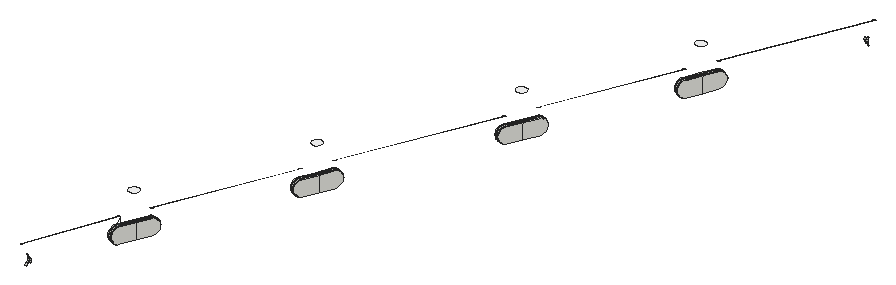
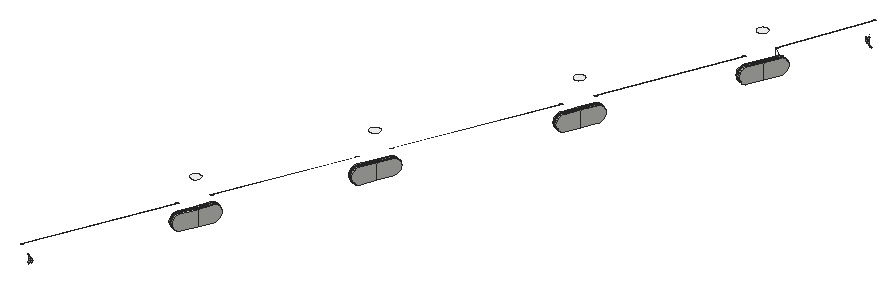
# SketchUp Ruby script. Lengths in inches.
U = 1.inch
M = Sketchup.active_model
def pt(a) = Geom::Point3d.new(a.map { |v| v * U })
def face(e, loops, mat)
  f = e.add_face(loops[0].map { |a| pt(a) })
  loops[1..].each { |l| e.add_face(l.map { |a| pt(a) }).erase! }
  f.material = f.back_material = mat if mat
  f
end
# faces: each face lists its corners as indices into pts; further lists are holes
def faces(e, pts, list, mat = nil) = list.each { |f| face(e, (f[0].is_a?(Array) ? f : [f]).map { |l| l.map { |i| pts[i] } }, mat) }
# xy, xz, yz: faces in a plane at the given z, y or x. An outline is a flat list of corners, or four numbers for a rectangle; further outlines are holes
def ring(l) = l.size == 4 ? [[l[0], l[1]], [l[2], l[1]], [l[2], l[3]], [l[0], l[3]]] : l.each_slice(2).to_a
def flat(e, list, mat, &to3) = list.each { |f| face(e, (f[0].is_a?(Array) ? f : [f]).map { |l| ring(l).map { |u, v| to3.(u, v) } }, mat) }
def xy(e, z, list, mat = nil) = flat(e, list, mat) { |x, y| [x, y, z] }
def xz(e, y, list, mat = nil) = flat(e, list, mat) { |x, z| [x, y, z] }
def yz(e, x, list, mat = nil) = flat(e, list, mat) { |y, z| [x, y, z] }
def lines(e, pts, list) = list.each { |a, b| e.add_line(pt(pts[a]), pt(pts[b])) }
# prism: a flat outline (further loops are holes) pulled along v
def prism(e, loops, v, mat = nil)
  f = face(e, loops, mat); d = Geom::Vector3d.new(v.map { |x| x * U })
  f.pushpull(f.normal.samedirection?(d) ? d.length : -d.length)
end
def box(e, o, s, mat = nil) = prism(e, [[o, [o[0] + s[0], o[1], o[2]], [o[0] + s[0], o[1] + s[1], o[2]], [o[0], o[1] + s[1], o[2]]]], [0, 0, s[2]], mat)
def at(x, y, z, deg = 0) = Geom::Transformation.translation(pt([x, y, z])) * Geom::Transformation.rotation(ORIGIN, Z_AXIS, deg.degrees)
def axes(o, x, y, z) = Geom::Transformation.new([*x, 0, *y, 0, *z, 0, *pt(o).to_a, 1])
def part(name) = M.definitions.add(name)
# library, detail: a bought-in or finely detailed component or shape, given as its bounding box
def library(name, o, s) = part(name).tap { |d| box(d.entities, o, s) }
def detail(e, o, s) = box(e.add_group.entities, o, s)
def put(e, d, t, mat = nil) = e.add_instance(d, t).tap { |i| i.material = mat if mat }
def group(e, t, mat = nil) = e.add_group.tap { |g| g.transformation = t; g.material = mat if mat }.entities
root = M.entities
M.materials.add("Glass_Safety_01").color = [204, 235, 244]
M.materials["Glass_Safety_01"].alpha = 0.1
M.materials.add("[Color_000]").color = [255, 255, 255]
xy(root,351.283,[[888.84,639.54,888.584,639.641,888.672,639.866,889.306,641.468,889.558,641.358],[888.4,639.713,888.144,639.814,888.868,641.645,889.124,641.544,888.489,639.938],[889.558,641.358,889.306,641.468,889.307,641.472,889.563,641.37,889.561,641.364],[889.563,641.37,889.307,641.472,890.092,643.273,890.344,643.163],[889.125,641.547,888.873,641.657,889.659,643.462,889.911,643.352],
  [897.674,659.993,897.421,660.103,897.491,660.262,898.207,661.907,898.46,661.797],[897.241,660.181,896.988,660.291,897.774,662.096,898.027,661.986,897.31,660.341],[898.46,661.797,898.207,661.907,898.994,663.712,899.246,663.602],[898.027,661.986,897.774,662.096,898.56,663.901,898.813,663.791],[907.619,682.827,907.367,682.937,907.429,683.08,908.153,684.742,908.405,684.632],
  [907.186,683.016,906.933,683.126,907.719,684.93,907.972,684.82,907.248,683.158],[908.405,684.632,908.153,684.742,908.939,686.547,909.191,686.436],[907.972,684.82,907.719,684.93,908.505,686.735,908.758,686.625],[916.339,702.848,916.086,702.958,916.157,703.12,916.872,704.763,917.125,704.653],[915.906,703.036,915.653,703.146,916.439,704.951,916.692,704.841,915.977,703.199],
  [917.125,704.653,916.872,704.763,917.658,706.567,917.911,706.457],[916.692,704.841,916.439,704.951,917.225,706.756,917.478,706.646]])
xy(root,351.362,[[888.728,640.007,888.545,640.079,889.124,641.544,889.215,641.508,889.306,641.468],[889.306,641.468,889.215,641.508,889.307,641.472,889.306,641.47],[889.307,641.472,889.215,641.508,889.125,641.547,889.754,642.991,889.935,642.912],[897.579,660.464,897.398,660.542,898.027,661.986,898.207,661.907],[898.207,661.907,898.027,661.986,898.656,663.43,898.836,663.351],
  [907.524,683.298,907.343,683.377,907.972,684.82,908.153,684.742],[908.153,684.742,907.972,684.82,908.601,686.264,908.781,686.186],[916.243,703.319,916.063,703.397,916.692,704.841,916.872,704.763],[916.872,704.763,916.692,704.841,917.321,706.285,917.501,706.206]],"Glass_Safety_01")
xy(root,353.33,[[888.728,640.007,889.306,641.468,889.215,641.508,889.124,641.544,888.545,640.079],[889.306,641.468,889.306,641.47,889.307,641.472,889.215,641.508],[889.307,641.472,889.935,642.912,889.754,642.991,889.125,641.547,889.215,641.508],[897.579,660.464,898.207,661.907,898.027,661.986,897.398,660.542],[898.207,661.907,898.836,663.351,898.656,663.43,898.027,661.986],
  [907.524,683.298,908.153,684.742,907.972,684.82,907.343,683.377],[908.153,684.742,908.781,686.186,908.601,686.264,907.972,684.82],[916.243,703.319,916.872,704.763,916.692,704.841,916.063,703.397],[916.872,704.763,917.501,706.206,917.321,706.285,916.692,704.841]],"Glass_Safety_01")
xy(root,353.409,[[888.84,639.54,889.558,641.358,889.306,641.468,888.672,639.866,888.584,639.641],[888.4,639.713,888.489,639.938,889.124,641.544,888.868,641.645,888.144,639.814],[889.558,641.358,889.561,641.364,889.563,641.37,889.307,641.472,889.306,641.468],[889.563,641.37,890.344,643.163,890.092,643.273,889.307,641.472],[889.125,641.547,889.911,643.352,889.659,643.462,888.873,641.657],
  [897.674,659.993,898.46,661.797,898.207,661.907,897.491,660.262,897.421,660.103],[897.241,660.181,897.31,660.341,898.027,661.986,897.774,662.096,896.988,660.291],[898.46,661.797,899.246,663.602,898.994,663.712,898.207,661.907],[898.027,661.986,898.813,663.791,898.56,663.901,897.774,662.096],[907.619,682.827,908.405,684.632,908.153,684.742,907.429,683.08,907.367,682.937],
  [907.186,683.016,907.248,683.158,907.972,684.82,907.719,684.93,906.933,683.126],[908.405,684.632,909.191,686.436,908.939,686.547,908.153,684.742],[907.972,684.82,908.758,686.625,908.505,686.735,907.719,684.93],[916.339,702.848,917.125,704.653,916.872,704.763,916.157,703.12,916.086,702.958],[915.906,703.036,915.977,703.199,916.692,704.841,916.439,704.951,915.653,703.146],
  [917.125,704.653,917.911,706.457,917.658,706.567,916.872,704.763],[916.692,704.841,917.478,706.646,917.225,706.756,916.439,704.951]])
xy(root,354.511,[[884.14,628.396,888.489,639.938,883.957,628.468],[884.14,628.396,888.672,639.866,888.489,639.938],[890.092,643.273,897.31,660.341,889.911,643.352],[890.092,643.273,897.491,660.262,897.31,660.341],[898.994,663.712,907.248,683.158,898.813,663.791],
  [898.994,663.712,907.429,683.08,907.248,683.158],[908.939,686.547,915.977,703.199,908.758,686.625],[908.939,686.547,916.157,703.12,915.977,703.199],[917.658,706.567,925.204,724.386,917.478,706.646],[917.658,706.567,925.385,724.307,925.204,724.386]],"Glass_Safety_01")
xy(root,357.267,[[889.26,640.879,889.422,640.912,889.569,640.986,889.692,641.095,889.782,641.233,889.834,641.389,889.844,641.553,889.811,641.714,889.737,641.861,889.628,641.984,889.491,642.074,889.335,642.126,889.17,642.136,889.009,642.103,888.862,642.029,888.739,641.92,888.649,641.783,888.597,641.627,888.587,641.463,888.62,641.302,888.694,641.155,888.803,641.032,888.94,640.941,889.096,640.889],[898.162,661.318,898.323,661.351,898.47,661.425,898.593,661.534,898.684,661.672,898.736,661.828,898.746,661.992,898.712,662.153,898.639,662.3,898.53,662.423,898.392,662.513,898.236,662.565,898.072,662.575,897.911,662.542,897.764,662.468,897.641,662.359,897.551,662.222,897.499,662.066,897.489,661.902,897.522,661.741,897.596,661.594,897.705,661.471,897.842,661.38,897.998,661.328],[908.107,684.153,908.268,684.186,908.415,684.259,908.538,684.369,908.629,684.506,908.681,684.662,908.691,684.826,908.658,684.987,908.584,685.134,908.475,685.257,908.337,685.348,908.181,685.4,908.017,685.409,907.856,685.376,907.709,685.303,907.586,685.194,907.496,685.056,907.444,684.9,907.434,684.736,907.467,684.575,907.541,684.428,907.65,684.305,907.787,684.214,907.943,684.163],[916.827,704.174,916.988,704.207,917.135,704.28,917.258,704.389,917.349,704.527,917.4,704.683,917.41,704.847,917.377,705.008,917.304,705.155,917.194,705.278,917.057,705.368,916.901,705.42,916.737,705.43,916.576,705.397,916.429,705.323,916.306,705.214,916.215,705.077,916.163,704.921,916.154,704.757,916.187,704.596,916.26,704.449,916.37,704.326,916.507,704.235,916.663,704.183]],"[Color_000]")
p = [[888.84,639.54,351.283],[889.558,641.358,351.283],[889.558,641.358,353.409],[888.84,639.54,353.409],[888.739,639.284,353.373],[888.644,639.045,353.267],
  [888.564,638.84,353.098],[888.501,638.683,352.877],[888.462,638.585,352.621],[888.449,638.551,352.346],[888.462,638.585,352.071],[888.501,638.683,351.814],
  [888.564,638.84,351.594],[888.644,639.045,351.425],[888.739,639.284,351.319],[888.4,639.713,351.283],[888.489,639.938,351.283],[888.489,639.938,353.409],
  [888.4,639.713,353.409],[888.299,639.457,353.373],[888.205,639.219,353.267],[888.124,639.014,353.098],[888.062,638.857,352.877],[888.023,638.758,352.621],
  [888.01,638.725,352.346],[888.023,638.758,352.071],[888.062,638.857,351.814],[888.124,639.014,351.594],[888.205,639.219,351.425],[888.299,639.457,351.319],
  [888.433,639.26,353.317],[888.202,638.675,352.163],[888.206,638.686,352.071],[888.245,638.785,351.814],[888.307,638.942,351.594],[888.388,639.147,351.425],
  [888.482,639.385,351.319],[888.584,639.641,351.283],[888.672,639.866,351.283],[888.672,639.866,353.409],[888.672,639.866,354.511],[889.306,641.468,353.409],
  [889.306,641.468,353.33],[889.306,641.468,351.362],[889.306,641.468,351.283],[888.193,638.652,352.346],[888.206,638.686,352.621],[888.245,638.785,352.877],
  [888.307,638.942,353.098],[888.388,639.147,353.267],[888.482,639.385,353.373],[888.584,639.641,353.409],[888.144,639.814,353.409],[888.868,641.645,353.409],
  [888.868,641.645,351.283],[888.144,639.814,351.283],[888.043,639.559,351.319],[887.949,639.32,351.425],[887.868,639.115,351.594],[887.806,638.958,351.814],
  [887.767,638.86,352.071],[887.753,638.826,352.346],[887.767,638.86,352.621],[887.806,638.958,352.877],[887.868,639.115,353.098],[887.949,639.32,353.267],
  [888.043,639.559,353.373],[889.124,641.544,353.409],[889.124,641.544,351.283],[889.124,641.544,351.362],[888.545,640.079,351.362],[888.545,640.079,353.33],
  [889.124,641.544,353.33],[889.307,641.472,351.283],[889.307,641.472,351.362],[889.307,641.472,353.33],[889.307,641.472,353.409],[889.563,641.37,353.409],
  [889.563,641.37,351.283],[889.561,641.364,353.409],[889.561,641.364,351.283],[890.344,643.163,351.283],[890.454,643.415,351.319],[890.557,643.65,351.425],
  [890.645,643.852,351.594],[890.712,644.007,351.814],[890.754,644.105,352.071],[890.769,644.138,352.346],[890.754,644.105,352.621],[890.712,644.007,352.877],
  [890.645,643.852,353.098],[890.557,643.65,353.267],[890.454,643.415,353.373],[890.344,643.163,353.409],[889.125,641.547,351.283],[889.125,641.547,351.362],
  [889.125,641.547,353.33],[889.125,641.547,353.409],[888.873,641.657,353.409],[888.873,641.657,351.283],[889.911,643.352,351.283],[889.911,643.352,353.409],
  [889.754,642.991,353.33],[889.754,642.991,351.362],[890.092,643.273,353.409],[890.202,643.525,353.373],[890.304,643.76,353.267],[890.392,643.962,353.098],
  [890.459,644.117,352.877],[890.502,644.215,352.621],[890.516,644.248,352.346],[890.502,644.215,352.071],[890.459,644.117,351.814],[890.392,643.962,351.594],
  [890.304,643.76,351.425],[890.202,643.525,351.319],[890.092,643.273,351.283],[889.659,643.462,353.409],[889.768,643.714,353.373],[889.871,643.949,353.267],
  [889.959,644.151,353.098],[890.026,644.306,352.877],[890.069,644.403,352.621],[890.083,644.436,352.346],[890.069,644.403,352.071],[890.026,644.306,351.814],
  [889.959,644.151,351.594],[889.871,643.949,351.425],[889.768,643.714,351.319],[889.659,643.462,351.283],[890.021,643.604,351.319],[890.021,643.604,353.373],
  [890.123,643.839,353.267],[890.211,644.041,353.098],[890.279,644.196,352.877],[890.321,644.293,352.621],[890.336,644.326,352.346],[890.321,644.293,352.071],
  [890.279,644.196,351.814],[890.211,644.041,351.594],[890.123,643.839,351.425],[898.46,661.797,353.409],[897.674,659.993,353.409],[897.564,659.74,353.373],
  [897.462,659.505,353.267],[897.374,659.303,353.098],[897.307,659.149,352.877],[897.264,659.051,352.621],[897.25,659.018,352.346],[897.264,659.051,352.071],
  [897.307,659.149,351.814],[897.374,659.303,351.594],[897.462,659.505,351.425],[897.564,659.74,351.319],[897.674,659.993,351.283],[898.46,661.797,351.283],
  [897.421,660.103,353.409],[897.491,660.262,353.409],[897.491,660.262,351.283],[897.421,660.103,351.283],[897.312,659.85,351.319],[897.209,659.615,351.425],
  [897.121,659.414,351.594],[897.054,659.259,351.814],[897.011,659.161,352.071],[896.997,659.128,352.346],[897.011,659.161,352.621],[897.054,659.259,352.877],
  [897.121,659.414,353.098],[897.209,659.615,353.267],[897.312,659.85,353.373],[897.241,660.181,351.283],[897.31,660.341,351.283],[897.31,660.341,353.409],
  [897.241,660.181,353.409],[897.131,659.929,353.373],[897.029,659.694,353.267],[896.941,659.492,353.098],[896.873,659.337,352.877],[896.831,659.24,352.621],
  [896.817,659.207,352.346],[896.831,659.24,352.071],[896.873,659.337,351.814],[896.941,659.492,351.594],[897.029,659.694,351.425],[897.131,659.929,351.319],
  [896.988,660.291,353.409],[897.774,662.096,353.409],[897.774,662.096,351.283],[896.988,660.291,351.283],[896.878,660.039,351.319],[896.776,659.804,351.425],
  [896.688,659.602,351.594],[896.621,659.447,351.814],[896.578,659.35,352.071],[896.564,659.317,352.346],[896.578,659.35,352.621],[896.621,659.447,352.877],
  [896.688,659.602,353.098],[896.776,659.804,353.267],[896.878,660.039,353.373],[898.027,661.986,353.409],[898.027,661.986,351.283],[898.027,661.986,351.362],
  [897.398,660.542,351.362],[897.398,660.542,353.33],[898.027,661.986,353.33],[898.207,661.907,351.283],[898.207,661.907,353.409],[898.207,661.907,353.33],
  [897.579,660.464,353.33],[897.579,660.464,351.362],[898.207,661.907,351.362],[899.246,663.602,353.409],[899.246,663.602,351.283],[899.356,663.854,351.319],
  [899.458,664.089,351.425],[899.546,664.291,351.594],[899.614,664.446,351.814],[899.656,664.543,352.071],[899.671,664.577,352.346],[899.656,664.543,352.621],
  [899.614,664.446,352.877],[899.546,664.291,353.098],[899.458,664.089,353.267],[899.356,663.854,353.373],[898.994,663.712,353.409],[898.994,663.712,351.283],
  [898.836,663.351,351.362],[898.836,663.351,353.33],[898.813,663.791,351.283],[898.813,663.791,353.409],[898.656,663.43,353.33],[898.656,663.43,351.362],
  [898.56,663.901,353.409],[898.67,664.153,353.373],[898.773,664.388,353.267],[898.86,664.59,353.098],[898.928,664.745,352.877],[898.97,664.842,352.621],
  [898.985,664.875,352.346],[898.97,664.842,352.071],[898.928,664.745,351.814],[898.86,664.59,351.594],[898.773,664.388,351.425],[898.67,664.153,351.319],
  [898.56,663.901,351.283],[899.103,663.964,351.319],[899.206,664.199,351.425],[899.294,664.401,351.594],[899.361,664.556,351.814],[899.403,664.654,352.071],
  [899.418,664.687,352.346],[899.403,664.654,352.621],[899.361,664.556,352.877],[899.294,664.401,353.098],[899.206,664.199,353.267],[899.103,663.964,353.373],
  [898.923,664.043,351.319],[898.923,664.043,353.373],[899.025,664.278,353.267],[899.113,664.48,353.098],[899.181,664.635,352.877],[899.223,664.732,352.621],
  [899.237,664.765,352.346],[899.223,664.732,352.071],[899.181,664.635,351.814],[899.113,664.48,351.594],[899.025,664.278,351.425],[908.405,684.632,353.409],
  [907.619,682.827,353.409],[907.509,682.575,353.373],[907.407,682.34,353.267],[907.319,682.138,353.098],[907.252,681.983,352.877],[907.209,681.886,352.621],
  [907.195,681.852,352.346],[907.209,681.886,352.071],[907.252,681.983,351.814],[907.319,682.138,351.594],[907.407,682.34,351.425],[907.509,682.575,351.319],
  [907.619,682.827,351.283],[908.405,684.632,351.283],[907.186,683.016,351.283],[907.248,683.158,351.283],[907.248,683.158,353.409],[907.186,683.016,353.409],
  [907.076,682.763,353.373],[906.974,682.528,353.267],[906.886,682.326,353.098],[906.818,682.172,352.877],[906.776,682.074,352.621],[906.762,682.041,352.346],
  [906.776,682.074,352.071],[906.818,682.172,351.814],[906.886,682.326,351.594],[906.974,682.528,351.425],[907.076,682.763,351.319],[907.367,682.937,353.409],
  [907.429,683.08,353.409],[907.429,683.08,351.283],[907.367,682.937,351.283],[907.257,682.685,351.319],[907.154,682.45,351.425],[907.066,682.248,351.594],
  [906.999,682.093,351.814],[906.957,681.996,352.071],[906.942,681.962,352.346],[906.957,681.996,352.621],[906.999,682.093,352.877],[907.066,682.248,353.098],
  [907.154,682.45,353.267],[907.257,682.685,353.373],[906.933,683.126,353.409],[907.719,684.93,353.409],[907.719,684.93,351.283],[906.933,683.126,351.283],
  [906.824,682.873,351.319],[906.721,682.638,351.425],[906.633,682.437,351.594],[906.566,682.282,351.814],[906.523,682.184,352.071],[906.509,682.151,352.346],
  [906.523,682.184,352.621],[906.566,682.282,352.877],[906.633,682.437,353.098],[906.721,682.638,353.267],[906.824,682.873,353.373],[908.153,684.742,351.283],
  [908.153,684.742,353.409],[908.153,684.742,353.33],[907.524,683.298,353.33],[907.524,683.298,351.362],[908.153,684.742,351.362],[907.972,684.82,353.409],
  [907.972,684.82,351.283],[907.972,684.82,351.362],[907.343,683.377,351.362],[907.343,683.377,353.33],[907.972,684.82,353.33],[909.191,686.436,353.409],
  [909.191,686.436,351.283],[909.301,686.689,351.319],[909.403,686.924,351.425],[909.491,687.126,351.594],[909.559,687.28,351.814],[909.601,687.378,352.071],
  [909.616,687.411,352.346],[909.601,687.378,352.621],[909.559,687.28,352.877],[909.491,687.126,353.098],[909.403,686.924,353.267],[909.301,686.689,353.373],
  [908.939,686.547,353.409],[908.939,686.547,351.283],[908.781,686.186,351.362],[908.781,686.186,353.33],[908.758,686.625,351.283],[908.758,686.625,353.409],
  [908.601,686.264,353.33],[908.601,686.264,351.362],[908.505,686.735,353.409],[908.615,686.987,353.373],[908.718,687.222,353.267],[908.806,687.424,353.098],
  [908.873,687.579,352.877],[908.915,687.677,352.621],[908.93,687.71,352.346],[908.915,687.677,352.071],[908.873,687.579,351.814],[908.806,687.424,351.594],
  [908.718,687.222,351.425],[908.615,686.987,351.319],[908.505,686.735,351.283],[909.048,686.799,351.319],[909.151,687.034,351.425],[909.239,687.236,351.594],
  [909.306,687.391,351.814],[909.349,687.488,352.071],[909.363,687.521,352.346],[909.349,687.488,352.621],[909.306,687.391,352.877],[909.239,687.236,353.098],
  [909.151,687.034,353.267],[909.048,686.799,353.373],[908.868,686.877,351.319],[908.868,686.877,353.373],[908.97,687.112,353.267],[909.058,687.314,353.098],
  [909.126,687.469,352.877],[909.168,687.567,352.621],[909.183,687.6,352.346],[909.168,687.567,352.071],[909.126,687.469,351.814],[909.058,687.314,351.594],
  [908.97,687.112,351.425],[917.125,704.653,353.409],[916.339,702.848,353.409],[916.229,702.596,353.373],[916.127,702.36,353.267],[916.039,702.159,353.098],
  [915.971,702.004,352.877],[915.929,701.906,352.621],[915.914,701.873,352.346],[915.929,701.906,352.071],[915.971,702.004,351.814],[916.039,702.159,351.594],
  [916.127,702.36,351.425],[916.229,702.596,351.319],[916.339,702.848,351.283],[917.125,704.653,351.283],[916.086,702.958,353.409],[916.157,703.12,353.409],
  [916.157,703.12,351.283],[916.086,702.958,351.283],[915.976,702.706,351.319],[915.874,702.47,351.425],[915.786,702.269,351.594],[915.719,702.114,351.814],
  [915.676,702.016,352.071],[915.662,701.983,352.346],[915.676,702.016,352.621],[915.719,702.114,352.877],[915.786,702.269,353.098],[915.874,702.47,353.267],
  [915.976,702.706,353.373],[915.906,703.036,351.283],[915.977,703.199,351.283],[915.977,703.199,353.409],[915.906,703.036,353.409],[915.796,702.784,353.373],
  [915.693,702.549,353.267],[915.606,702.347,353.098],[915.538,702.192,352.877],[915.496,702.095,352.621],[915.481,702.062,352.346],[915.496,702.095,352.071],
  [915.538,702.192,351.814],[915.606,702.347,351.594],[915.693,702.549,351.425],[915.796,702.784,351.319],[915.653,703.146,353.409],[916.439,704.951,353.409],
  [916.439,704.951,351.283],[915.653,703.146,351.283],[915.543,702.894,351.319],[915.441,702.659,351.425],[915.353,702.457,351.594],[915.285,702.302,351.814],
  [915.243,702.205,352.071],[915.229,702.172,352.346],[915.243,702.205,352.621],[915.285,702.302,352.877],[915.353,702.457,353.098],[915.441,702.659,353.267],
  [915.543,702.894,353.373],[916.872,704.763,351.283],[916.872,704.763,353.409],[916.872,704.763,353.33],[916.243,703.319,353.33],[916.243,703.319,351.362],
  [916.872,704.763,351.362],[916.692,704.841,353.409],[916.692,704.841,351.283],[916.692,704.841,351.362],[916.063,703.397,351.362],[916.063,703.397,353.33],
  [916.692,704.841,353.33],[917.911,706.457,353.409],[917.911,706.457,351.283],[918.021,706.71,351.319],[918.123,706.945,351.425],[918.211,707.146,351.594],
  [918.278,707.301,351.814],[918.321,707.399,352.071],[918.335,707.432,352.346],[918.321,707.399,352.621],[918.278,707.301,352.877],[918.211,707.146,353.098],
  [918.123,706.945,353.267],[918.021,706.71,353.373],[917.478,706.646,351.283],[917.478,706.646,353.409],[917.321,706.285,353.33],[917.321,706.285,351.362],
  [917.658,706.567,353.409],[917.658,706.567,351.283],[917.501,706.206,351.362],[917.501,706.206,353.33],[917.225,706.756,353.409],[917.335,707.008,353.373],
  [917.437,707.243,353.267],[917.525,707.445,353.098],[917.593,707.6,352.877],[917.635,707.697,352.621],[917.65,707.731,352.346],[917.635,707.697,352.071],
  [917.593,707.6,351.814],[917.525,707.445,351.594],[917.437,707.243,351.425],[917.335,707.008,351.319],[917.225,706.756,351.283],[917.768,706.82,351.319],
  [917.588,706.898,351.319],[917.588,706.898,353.373],[917.69,707.133,353.267],[917.778,707.335,353.098],[917.845,707.49,352.877],[917.888,707.587,352.621],
  [917.902,707.62,352.346],[917.888,707.587,352.071],[917.845,707.49,351.814],[917.778,707.335,351.594],[917.69,707.133,351.425],[917.87,707.055,351.425],
  [917.958,707.256,351.594],[918.026,707.411,351.814],[918.068,707.509,352.071],[918.083,707.542,352.346],[918.068,707.509,352.621],[918.026,707.411,352.877],
  [917.958,707.256,353.098],[917.87,707.055,353.267],[917.768,706.82,353.373],[888.728,640.007,351.362],[888.728,640.007,353.33],[889.215,641.508,353.33],
  [889.215,641.508,351.362],[889.306,641.47,351.362],[889.306,641.47,353.33],[889.935,642.912,353.33],[889.935,642.912,351.362],[884.295,629.324,351.814],
  [884.233,629.167,351.594],[883.977,629.268,351.594],[884.039,629.425,351.814],[884.334,629.423,352.071],[884.078,629.524,352.071],[924.908,723.212,352.071],
  [924.95,723.31,351.814],[925.203,723.2,351.814],[925.16,723.102,352.071],[884.517,629.35,352.071],[884.53,629.384,352.346],[884.787,629.283,352.346],
  [884.773,629.249,352.071],[884.347,629.456,352.346],[884.091,629.558,352.346],[924.893,723.179,352.346],[925.146,723.069,352.346],[924.727,723.291,352.071],
  [924.713,723.258,352.346],[924.46,723.368,352.346],[924.474,723.401,352.071],[884.517,629.35,352.621],[884.773,629.249,352.621],[884.334,629.423,352.621],
  [884.078,629.524,352.621],[924.908,723.212,352.621],[925.16,723.102,352.621],[924.727,723.291,352.621],[924.474,723.401,352.621],[884.295,629.324,352.877],
  [884.329,629.411,352.653],[884.039,629.425,352.877],[924.95,723.31,352.877],[925.203,723.2,352.877],[884.257,629.229,353.01]]
faces(root,p,[[0,1,2,3,4,5,6,7,8,9,10,11,12,13,14],[15,16,17,18,19,20,21,22,23,24,25,26,27,28,29],[39,41,42,43,44,38,37,36,35,34,33,32,31,45,46,47,48,49,30,50,51],[52,53,54,55,56,57,58,59,60,61,62,63,64,65,66],[35,36,14,13],[29,28,57,56],[36,37,0,14],[15,29,56,55],
  [67,17,16,68,69,70,71,72],[43,44,1,2,41,42],[73,74,75,76,77,78],[79,2,1,80,78,77],[79,2,1,80,78,81,82,83,84,85,86,87,88,89,90,91,92,93,77],[69,68,54,53,67,72],[94,95,96,97,98,99],[94,100,101,97,96,102,103,95],
  [73,44,43,42,41,76,75,74],[41,76,104,105,106,107,108,109,110,111,112,113,114,115,116,73,44,43,42],[98,117,118,119,120,121,122,123,124,125,126,127,128,129,99],[116,115,82,81],[130,100,129,128],[115,114,83,82],[140,130,128,127],[141,142,143,144,145,146,147,148,149,150,151,152,153,154,155],
  [156,157,158,159,160,161,162,163,164,165,166,167,168,169,170],[171,172,173,174,175,176,177,178,179,180,181,182,183,184,185],[186,187,188,189,190,191,192,193,194,195,196,197,198,199,200],[161,160,153,152],[185,184,191,190],[160,159,154,153],[171,185,190,189],[201,173,172,202,203,204,205,206],
  [207,158,157,208,209,210,211,212],[207,212,209,208,141,155],[213,141,155,214,215,216,217,218,219,220,221,222,223,224,225],[208,226,227,207,212,228,229,209],[203,202,188,187,201,206],[202,230,231,201,206,232,233,203],[187,234,235,236,237,238,239,240,241,242,243,244,245,246,188],[227,247,215,214],
  [258,230,246,245],[247,248,216,215],[268,258,245,244],[269,270,271,272,273,274,275,276,277,278,279,280,281,282,283],[284,285,286,287,288,289,290,291,292,293,294,295,296,297,298],[299,300,301,302,303,304,305,306,307,308,309,310,311,312,313],[314,315,316,317,318,319,320,321,322,323,324,325,326,327,328],[304,303,281,280],
  [298,297,319,318],[303,302,282,281],[284,298,318,317],[329,301,300,330,331,332,333,334],[335,286,285,336,337,338,339,340],[329,334,331,330,269,283],[341,269,283,342,343,344,345,346,347,348,349,350,351,352,353],[330,354,355,329,334,356,357,331],
  [337,336,316,315,335,340],[336,358,359,335,340,360,361,337],[315,362,363,364,365,366,367,368,369,370,371,372,373,374,316],[355,375,343,342],[386,358,374,373],[375,376,344,343],[396,386,373,372],[397,398,399,400,401,402,403,404,405,406,407,408,409,410,411],
  [412,413,414,415,416,417,418,419,420,421,422,423,424,425,426],[427,428,429,430,431,432,433,434,435,436,437,438,439,440,441],[442,443,444,445,446,447,448,449,450,451,452,453,454,455,456],[417,416,409,408],[441,440,447,446],[416,415,410,409],[427,441,446,445],[457,414,413,458,459,460,461,462],
  [463,429,428,464,465,466,467,468],[457,462,459,458,397,411],[469,397,411,470,471,472,473,474,475,476,477,478,479,480,481],[465,464,444,443,463,468],[464,482,483,463,468,484,485,465],[458,486,487,457,462,488,489,459],[443,490,491,492,493,494,495,496,497,498,499,500,501,502,444],[487,503,471,470],
  [504,482,502,501],[503,515,472,471],[514,504,501,500],[34,35,13,12],[28,27,58,57],[114,113,84,83],[139,140,127,126],[162,161,152,151],
  [184,183,192,191],[248,249,217,216],[267,268,244,243],[305,304,280,279],[297,296,320,319],[376,377,345,344],[395,396,372,371],[418,417,408,407],
  [440,439,448,447],[515,516,473,472],[513,514,500,499],[533,534,535,536],[33,34,12,11],[27,26,59,58],[113,112,85,84],[138,139,126,125],
  [163,162,151,150],[183,182,193,192],[249,250,218,217],[266,267,243,242],[306,305,279,278],[296,295,321,320],[377,378,346,345],[394,395,371,370],
  [419,418,407,406],[439,438,449,448],[516,517,474,473],[512,513,499,498],[537,533,536,538],[32,33,11,10],[26,25,60,59],[112,111,86,85],
  [137,138,125,124],[164,163,150,149],[182,181,194,193],[250,251,219,218],[265,266,242,241],[307,306,278,277],[295,294,322,321],[378,379,347,346],
  [393,394,370,369],[420,419,406,405],[438,437,450,449],[517,518,475,474],[511,512,498,497],[539,540,541,542],[543,544,545,546],[547,537,538,548],
  [45,31,32,10,9],[25,24,61,60],[111,110,87,86],[136,137,124,123],[165,164,149,148],[181,180,195,194],[251,252,220,219],[264,265,241,240],
  [308,307,277,276],[294,293,323,322],[379,380,348,347],[392,393,369,368],[421,420,405,404],[437,436,451,450],[518,519,476,475],[510,511,497,496],
  [549,539,542,550],[551,552,553,554],[544,555,556,545],[557,547,548,558],[46,45,9,8],[24,23,62,61],[110,109,88,87],[135,136,123,122],
  [166,165,148,147],[180,179,196,195],[252,253,221,220],[263,264,240,239],[309,308,276,275],[293,292,324,323],[380,381,349,348],[391,392,368,367],
  [422,421,404,403],[436,435,452,451],[519,520,477,476],[509,510,496,495],[559,549,550,560],[552,561,562,553],[563,564,557,558,565],[47,46,8,7],
  [23,22,63,62],[109,108,89,88],[134,135,122,121],[167,166,147,146],[179,178,197,196],[253,254,222,221],[262,263,239,238],[310,309,275,274],
  [292,291,325,324],[381,382,350,349],[390,391,367,366],[423,422,403,402],[435,434,453,452],[520,521,478,477],[508,509,495,494],[566,559,560,567],
  [48,47,7,6],[22,21,64,63],[108,107,90,89],[133,134,121,120],[168,167,146,145],[178,177,198,197],[254,255,223,222],[261,262,238,237],
  [311,310,274,273],[291,290,326,325],[382,383,351,350],[389,390,366,365],[424,423,402,401],[434,433,454,453],[521,522,479,478],[507,508,494,493],
  [49,48,6,5],[21,20,65,64],[107,106,91,90],[132,133,120,119],[169,168,145,144],[177,176,199,198],[255,256,224,223],[260,261,237,236],
  [312,311,273,272],[290,289,327,326],[383,384,352,351],[388,389,365,364],[425,424,401,400],[433,432,455,454],[522,523,480,479],[506,507,493,492],
  [50,30,49,5,4],[20,19,66,65],[106,105,92,91],[131,132,119,118],[170,169,144,143],[176,175,200,199],[256,257,225,224],[259,260,236,235],
  [313,312,272,271],[289,288,328,327],[384,385,353,352],[387,388,364,363],[426,425,400,399],[432,431,456,455],[523,524,481,480],[505,506,492,491],
  [51,50,4,3],[19,18,52,66],[105,104,93,92],[101,131,118,117],[156,170,143,142],[175,174,186,200],[257,226,213,225],[231,259,235,234],
  [299,313,271,270],[288,287,314,328],[385,354,341,353],[359,387,363,362],[412,426,399,398],[431,430,442,456],[524,486,469,481],[483,505,491,490]])
faces(root,p,[[30,31,32,33,34,35,36,37,38,39,40],[104,116,115,114,113,112,111,110,109,108,107,106,105],[100,101,131,132,133,134,135,136,137,138,139,140,130],[226,227,247,248,249,250,251,252,253,254,255,256,257],[230,231,259,260,261,262,263,264,265,266,267,268,258],[354,355,375,376,377,378,379,380,381,382,383,384,385],[358,359,387,388,389,390,391,392,393,394,395,396,386],[482,483,505,506,507,508,509,510,511,512,513,514,504],
  [486,487,503,515,516,517,518,519,520,521,522,523,524],[71,70,525,526],[525,43,42,526],[72,71,70,69],[72,527,528,69],[528,527,96,95],[102,96,95,103],[527,528,43,42],
  [74,528,527,75],[529,74,75,530,42,43],[531,75,74,532],[102,531,532,103],[205,204,211,210],[206,205,204,203],[210,209,212,211],[206,209,212,203],
  [209,229,228,212],[232,206,203,233],[229,228,233,232],[339,338,333,332],[332,331,334,333],[340,339,338,337],[340,331,334,337],[331,357,356,334],
  [360,340,337,361],[357,356,361,360],[467,466,461,460],[460,459,462,461],[468,467,466,465],[468,459,462,465],[484,468,465,485],[459,489,488,462],
  [489,488,485,484],[31,30,49,48,47,46,45],[564,568,563]],"Glass_Safety_01")
